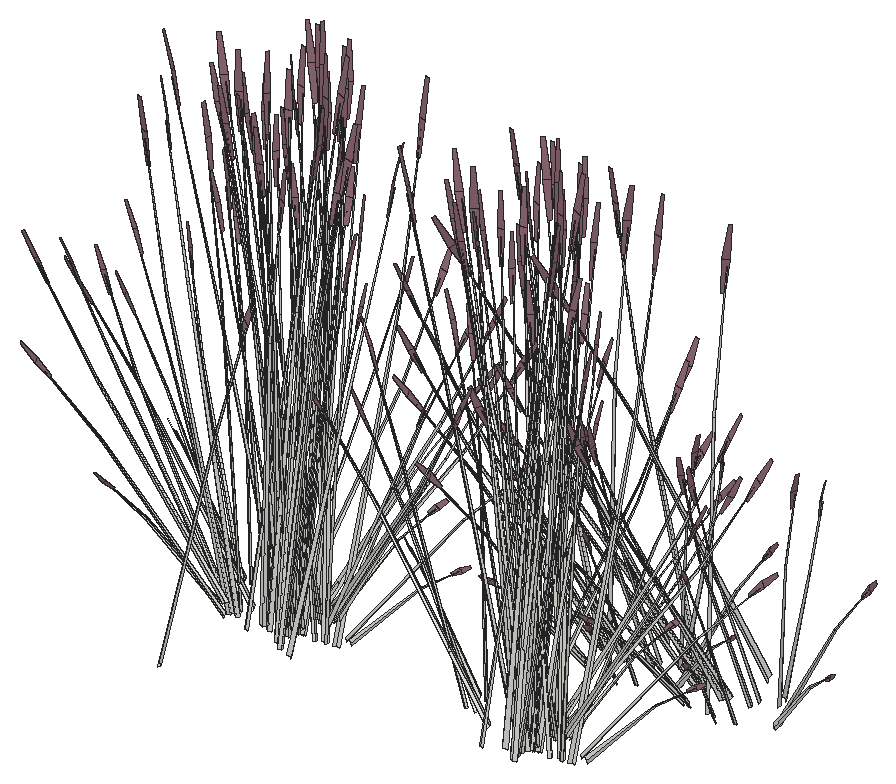
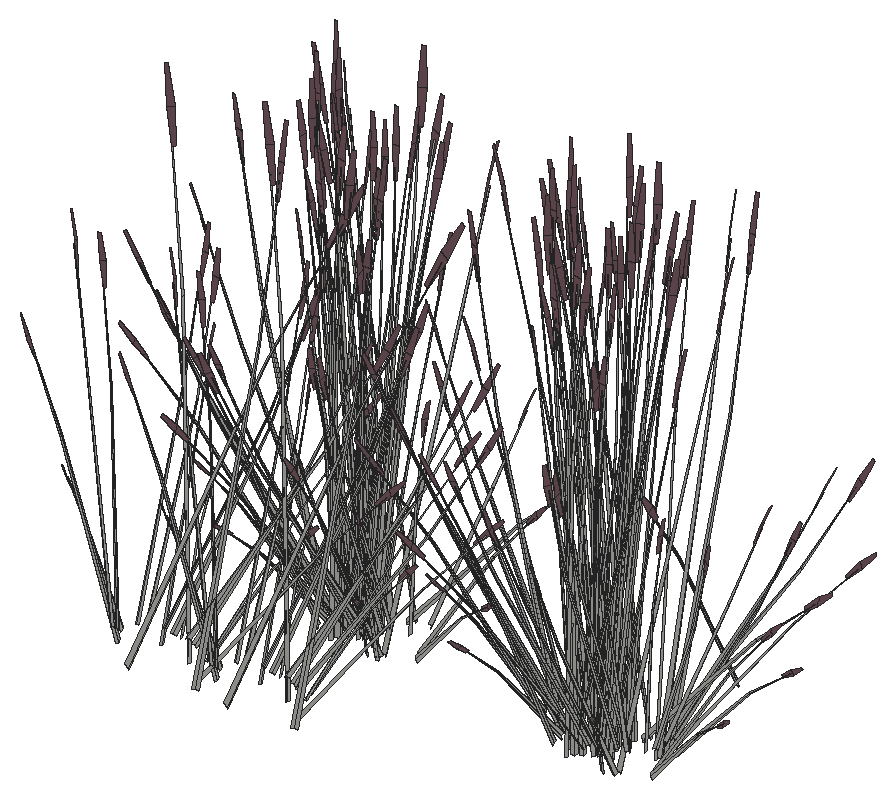
# SketchUp Ruby script. Lengths in inches.
U = 1.inch
M = Sketchup.active_model
def pt(a) = Geom::Point3d.new(a.map { |v| v * U })
def face(e, loops, mat)
  f = e.add_face(loops[0].map { |a| pt(a) })
  loops[1..].each { |l| e.add_face(l.map { |a| pt(a) }).erase! }
  f.material = f.back_material = mat if mat
  f
end
# faces: each face lists its corners as indices into pts; further lists are holes
def faces(e, pts, list, mat = nil) = list.each { |f| face(e, (f[0].is_a?(Array) ? f : [f]).map { |l| l.map { |i| pts[i] } }, mat) }
# xy, xz, yz: faces in a plane at the given z, y or x. An outline is a flat list of corners, or four numbers for a rectangle; further outlines are holes
def ring(l) = l.size == 4 ? [[l[0], l[1]], [l[2], l[1]], [l[2], l[3]], [l[0], l[3]]] : l.each_slice(2).to_a
def flat(e, list, mat, &to3) = list.each { |f| face(e, (f[0].is_a?(Array) ? f : [f]).map { |l| ring(l).map { |u, v| to3.(u, v) } }, mat) }
def xy(e, z, list, mat = nil) = flat(e, list, mat) { |x, y| [x, y, z] }
def xz(e, y, list, mat = nil) = flat(e, list, mat) { |x, z| [x, y, z] }
def yz(e, x, list, mat = nil) = flat(e, list, mat) { |y, z| [x, y, z] }
def lines(e, pts, list) = list.each { |a, b| e.add_line(pt(pts[a]), pt(pts[b])) }
# prism: a flat outline (further loops are holes) pulled along v
def prism(e, loops, v, mat = nil)
  f = face(e, loops, mat); d = Geom::Vector3d.new(v.map { |x| x * U })
  f.pushpull(f.normal.samedirection?(d) ? d.length : -d.length)
end
def box(e, o, s, mat = nil) = prism(e, [[o, [o[0] + s[0], o[1], o[2]], [o[0] + s[0], o[1] + s[1], o[2]], [o[0], o[1] + s[1], o[2]]]], [0, 0, s[2]], mat)
def at(x, y, z, deg = 0) = Geom::Transformation.translation(pt([x, y, z])) * Geom::Transformation.rotation(ORIGIN, Z_AXIS, deg.degrees)
def axes(o, x, y, z) = Geom::Transformation.new([*x, 0, *y, 0, *z, 0, *pt(o).to_a, 1])
def part(name) = M.definitions.add(name)
# library, detail: a bought-in or finely detailed component or shape, given as its bounding box
def library(name, o, s) = part(name).tap { |d| box(d.entities, o, s) }
def detail(e, o, s) = box(e.add_group.entities, o, s)
def put(e, d, t, mat = nil) = e.add_instance(d, t).tap { |i| i.material = mat if mat }
def group(e, t, mat = nil) = e.add_group.tap { |g| g.transformation = t; g.material = mat if mat }.entities
root = M.entities
M.materials.add("LightPink_Translucent").color = [144, 107, 117]
c1 = part("blade")
p = [[2.15,0.21,22],[0,0.17,0],[0.09,0.45,0],[2.18,0.31,22],[2.29,0.31,22],[0.38,0.45,0],
  [2.48,0.24,33],[2.49,0.24,33],[2.48,0.22,33]]
faces(c1.entities,p,[[0,1,2,3],[4,5,2,3],[6,3,4,7],[8,0,3,6]])
c2 = part("seeds")
p = [[0.3,-0.1,1.38],[-0.01,-0.03,1.59],[-0.01,-0.03,0.03],[0.14,-0.07,-0.07],[0.29,-0.03,3],[0.15,0.01,3.11]]
faces(c2.entities,p,[[0,1,2,3],[1,0,4,5]],"LightPink_Translucent")
c3 = part("blade with seeds")
put(c3.entities,c1,at(0,0,0))
put(c3.entities,c2,axes([2.4,0.25,30.99],[1.5799,-0.05474,1.17369],[-0.12525,1.92788,0.29478],[-0.07173,-0.02425,1.56792]))
put(root,c3,axes([68.36,54.11,46.98],[1.07686,-0.45739,-0.71045],[0.60013,0.94154,0.08574],[0.52031,-0.10696,1.00501]))
put(root,c3,axes([63.53,52.48,44.36],[-1.01611,0.93987,0.45755],[-1.20717,-0.82966,0.17955],[0.24496,-0.0938,1.58856]))
put(root,c3,axes([26.46,57.1,44.375],[-1.53239,0,0],[0,-1.1575,-0.51607],[0,-0.26363,1.63711]))
put(root,c3,axes([64.64,54.17,44.3],[-1.1399,-0.8914,-0.06131],[1.1406,-0.89194,0],[-0.03981,-0.03113,1.75571]))
put(root,c3,axes([26.72,55.03,44.59],[0.23927,0.28834,1.43002],[-0.55135,0.78376,-0.30754],[-0.56612,-0.18733,0.61141]))
put(root,c3,axes([61.77,50.93,44.47],[-0.35402,1.02926,0.17642],[-1.29548,-0.29127,0.35086],[0.22379,-0.00501,1.60407]))
put(root,c3,axes([28.39,42.73,45.36],[0.02693,-0.53464,1.54345],[1.21102,0.2824,0.21329],[-0.10493,0.5698,0.72882]))
put(root,c3,axes([64.48,52.08,44.62],[0.23642,-0.92427,0.1448],[1.15506,0.16044,-0.41347],[0.21021,0.09491,1.26744]))
put(root,c3,axes([27.71,54.77,46.98],[-1.22504,-0.02494,-0.71045],[0.08228,-1.05005,0.08574],[-0.51899,-0.11081,1.00501]))
put(root,c3,axes([62.48,54.27,44.36],[1.54892,0.2182,0.45755],[-0.31522,1.23236,0.17955],[-0.22636,-0.119,1.58856]))
put(root,c3,axes([63.98,52.32,44.72],[-0.73619,-0.86927,0.44739],[1.11511,-0.61213,-0.21531],[0.23824,0.10756,1.43643]))
put(root,c3,axes([61.65,56.24,44.47],[1.31687,-0.27488,0.17642],[0.32517,1.02297,0.35086],[-0.11745,-0.14905,1.60407]))
put(root,c3,axes([27.65,56.79,44.33],[-1.1399,0.87071,0.30756],[-1.1406,-0.86155,-0.36492],[-0.03981,-0.24727,1.64885]))
put(root,c3,axes([65.3,53.51,44.21],[1.37109,0,0],[0,1.07219,0],[0,0,1.78407]))
put(root,c3,axes([31.27,57.2,44.43],[1.3808,0.50196,0.24065],[-0.66454,1.04299,0.50002],[0,-0.24043,1.60543]))
put(root,c3,axes([65.6875,50.99,44.47],[-1.31687,0.27488,0.17642],[-0.32517,-1.02297,0.35086],[0.11745,0.14905,1.60407]))
put(root,c3,axes([27.3,54.99,46.68],[-0.88986,0.68603,-0.51099],[-0.77932,-0.72471,-0.3958],[-0.45212,-0.10438,0.97773]))
put(root,c3,axes([25.3,55.9,44.77],[0.78239,-0.07411,1.1486],[-0.49629,0.65296,0.84392],[-0.38663,-0.09795,0.25299]))
put(root,c3,axes([30.83,56.5,44.72],[-1.33077,0.06393,0.44739],[-0.12035,-1.06125,-0.21531],[0.23824,-0.10756,1.43643]))
put(root,c3,axes([27.39,57.27,44.48],[0,1.03566,0.49651],[-1.37109,0,0],[0,-0.23588,1.57504]))
put(root,c3,axes([64.86,52.96,44.38],[-1.54892,-0.2182,0.49198],[0.31522,-1.23236,0.19306],[0.22636,0.119,1.70813]))
put(root,c3,axes([37.02,57.51,46.68],[0.332,-0.94205,-0.51099],[1.13828,0.3229,-0.3958],[0.45829,-0.08638,0.97773]))
put(root,c3,axes([63.62,56,44.2],[-0.39985,-0.89288,0],[1.1418,-0.31268,0],[0,0,1.54371]))
put(root,c3,axes([35.22,53.67,44.375],[0.7662,-1.03778,0],[1.28187,0.57875,-0.51607],[0.29196,0.13181,1.63711]))
put(root,c3,axes([62.86,55.15,44.62],[-0.23642,0.92427,0.1448],[-1.15506,-0.16044,-0.41347],[-0.21021,-0.09491,1.26744]))
put(root,c3,axes([30.78,56.88,44.36],[0.53281,1.15808,0.45755],[-1.52239,0.4027,0.17955],[0.01861,-0.2128,1.58856]))
put(root,c3,axes([65.5625,56.3,44.47],[0.35402,-1.02926,0.17642],[1.29548,0.29127,0.35086],[-0.22379,0.00501,1.60407]))
put(root,c3,axes([65.27,53.96,44.21],[0.85545,0.66896,0],[-0.85545,0.66896,0],[0,0,1.69266]))
put(root,c3,axes([30.51,57.8,44.72],[-0.59459,0.93321,0.44739],[-1.23546,-0.44912,-0.21531],[0,-0.21512,1.43643]))
put(root,c3,axes([60.41,52.71,45.34],[0.34834,-0.14982,1.77064],[0.12012,1.04605,0.13857],[-0.75452,0.1388,0.63284]))
put(root,c3,axes([67.59,53.67,44.47],[-0.96285,-0.75439,0.17642],[0.97031,-0.7317,0.35086],[-0.10634,0.15406,1.60407]))
put(root,c3,axes([32.7,56.98,44.21],[0,-1.19833,0],[1.53239,0,0],[0,0,1.79456]))
put(root,c3,axes([71.4375,54.36,44.77],[-0.75718,0.17097,1.1486],[0.35641,-0.70661,0.84392],[0.40168,0.04835,0.25299]))
put(root,c3,axes([34.56,54.21,44.48],[-1.14694,-0.51783,0.49651],[0.68554,-0.92854,0],[0.26122,0.11794,1.57504]))
put(root,c3,axes([36.8,57.85,46.98],[1.07686,-0.45739,-0.71045],[0.60013,0.94154,0.08574],[0.52031,-0.10696,1.00501]))
put(root,c3,axes([63.34,56.41,44.2],[-1.23546,-0.46496,0],[0.59459,-0.96613,0],[0,0,1.62707]))
put(root,c3,axes([61.22,56.77,44.48],[1.14694,0.51783,0.49651],[-0.68554,0.92854,0],[-0.26122,-0.11794,1.57504]))
put(root,c3,axes([31.97,56.23,44.36],[-1.01611,0.93987,0.45755],[-1.20717,-0.82966,0.17955],[0.24496,-0.0938,1.58856]))
put(root,c3,axes([65.26,53.18,44.72],[0.59459,-0.93321,0.44739],[1.23546,0.44912,-0.21531],[0,0.21512,1.43643]))
put(root,c3,axes([33.08,57.91,44.3],[-1.1399,-0.8914,-0.06131],[1.1406,-0.89194,0],[-0.03981,-0.03113,1.75571]))
put(root,c3,axes([30.21,54.68,44.47],[-0.35402,1.02926,0.17642],[-1.29548,-0.29127,0.35086],[0.22379,-0.00501,1.60407]))
put(root,c3,axes([65.03,53.72,44.29],[0,1.19774,-0.05637],[-1.53239,0,0],[0,0.03764,1.79368]))
put(root,c3,axes([58,53.28,46.68],[-0.332,0.94205,-0.51099],[-1.13828,-0.3229,-0.3958],[-0.45829,0.08638,0.97773]))
put(root,c3,axes([32.91,55.82,44.62],[0.23642,-0.92427,0.1448],[1.15506,0.16044,-0.41347],[0.21021,0.09491,1.26744]))
put(root,c3,axes([60.56,57.31,44.375],[-0.7662,1.03778,0],[-1.28187,-0.57875,-0.51607],[-0.29196,-0.13181,1.63711]))
put(root,c3,axes([30.92,58.02,44.36],[1.54892,0.2182,0.45755],[-0.31522,1.23236,0.17955],[-0.22636,-0.119,1.58856]))
put(root,c3,axes([68.38,53.7,44.48],[0,-1.03566,0.49651],[1.37109,0,0],[0,0.23588,1.57504]))
put(root,c3,axes([64.94,54.48,44.72],[1.33077,-0.06393,0.44739],[0.12035,1.06125,-0.21531],[-0.23824,0.10756,1.43643]))
put(root,c3,axes([65.77,53.4,44.62],[1.1418,-0.30203,0.1448],[0.39985,0.86246,-0.41347],[0,0.18981,1.26744]))
put(root,c3,axes([32.42,56.07,44.72],[-0.73619,-0.86927,0.44739],[1.11511,-0.61213,-0.21531],[0.23824,0.10756,1.43643]))
put(root,c3,axes([70.02,55.5,44.59],[-0.29514,-0.25472,1.43002],[0.38401,-0.84262,-0.30754],[0.59714,0.11414,0.61141]))
put(root,c3,axes([30.08,59.99,44.47],[1.31687,-0.27488,0.17642],[0.32517,1.02297,0.35086],[-0.11745,-0.14905,1.60407]))
put(root,c3,axes([37.71,57.94,46.53],[1.01846,0.28891,-0.35414],[-0.29705,0.84289,0.4572],[0.41005,-0.07729,0.87481]))
put(root,c3,axes([64.74,56.42,44.2],[1.23546,0.46496,0],[-0.59459,0.96613,0],[0,0,1.74954]))
put(root,c3,axes([25.74,56.59,46.53],[-1.01846,-0.28891,-0.35414],[0.29705,-0.84289,0.4572],[-0.41005,0.07729,0.87481]))
put(root,c3,axes([33.74,57.25,44.21],[1.37109,0,0],[0,1.07219,0],[0,0,1.78407]))
put(root,c3,axes([34.125,54.73,44.47],[-1.31687,0.27488,0.17642],[-0.32517,-1.02297,0.35086],[0.11745,0.14905,1.60407]))
put(root,c3,axes([65.23,57.45,44.19],[-0.75665,-1.04141,-0.05142],[1.28187,-0.57875,0.51607],[-0.31588,0.09915,1.6363]))
put(root,c3,axes([64.97,54.93,44.62],[0.90538,0.62224,0.1448],[-0.75521,0.70202,-0.41347],[-0.21021,0.09491,1.26744]))
put(root,c3,axes([67.31,56.01,46.98],[1.22504,0.02494,-0.71045],[-0.08228,1.05005,0.08574],[0.51899,0.11081,1.00501]))
put(root,c3,axes([33.29,56.7,44.38],[-1.54892,-0.2182,0.49198],[0.31522,-1.23236,0.19306],[0.22636,0.119,1.70813]))
put(root,c3,axes([32.06,59.75,44.2],[-0.39985,-0.89288,0],[1.1418,-0.31268,0],[0,0,1.54371]))
put(root,c3,axes([65.93,56.85,44.48],[1.14694,-0.51783,0.49651],[0.68554,0.92854,0],[-0.26122,0.11794,1.57504]))
put(root,c3,axes([31.3,58.9,44.62],[-0.23642,0.92427,0.1448],[-1.15506,-0.16044,-0.41347],[-0.21021,-0.09491,1.26744]))
put(root,c3,axes([64.3,56.03,44.29],[0.53281,1.18979,-0.06012],[-1.52239,0.41691,0],[0.01861,0.04155,1.72173]))
put(root,c3,axes([34,60.04,44.47],[0.35402,-1.02926,0.17642],[1.29548,0.29127,0.35086],[-0.22379,0.00501,1.60407]))
put(root,c3,axes([56.64,55.49,44.59],[0.42589,0.08502,1.43002],[0.2745,0.86839,-0.30754],[-0.57851,0.16255,0.61141]))
put(root,c3,axes([33.71,57.71,44.21],[0.85545,0.66896,0],[-0.85545,0.66896,0],[0,0,1.69266]))
put(root,c3,axes([69.31,53.88,44.375],[1.53239,0,0],[0,1.1575,-0.51607],[0,0.26363,1.63711]))
put(root,c3,axes([28.84,56.45,45.34],[0.34834,-0.14982,1.77064],[0.12012,1.04605,0.13857],[-0.75452,0.1388,0.63284]))
put(root,c3,axes([36.02,57.42,44.47],[-0.96285,-0.75439,0.17642],[0.97031,-0.7317,0.35086],[-0.10634,0.15406,1.60407]))
put(root,c3,axes([68.7,54.47,44.2],[-1.53164,-0.00828,-0.04976],[0,-1.1575,0.49943],[-0.04813,0.2635,1.58352]))
put(root,c3,axes([39.875,58.11,44.77],[-0.75718,0.17097,1.1486],[0.35641,-0.70661,0.84392],[0.40168,0.04835,0.25299]))
put(root,c3,axes([55.75,57.31,44.77],[0.51072,-0.46938,1.1486],[0.20153,0.74307,0.84392],[-0.36908,0.13305,0.25299]))
put(root,c3,axes([68.05,56.44,46.53],[0.69728,0.64842,-0.35414],[-0.79619,0.61382,0.4572],[0.40453,0.09339,0.87481]))
put(root,c3,axes([31.78,60.15,44.2],[-1.23546,-0.46496,0],[0.59459,-0.96613,0],[0,0,1.62707]))
put(root,c3,axes([29.65,60.51,44.48],[1.14694,0.51783,0.49651],[-0.68554,0.92854,0],[-0.26122,-0.11794,1.57504]))
put(root,c3,axes([33.7,56.93,44.72],[0.59459,-0.93321,0.44739],[1.23546,0.44912,-0.21531],[0,0.21512,1.43643]))
put(root,c3,axes([33.47,57.46,44.29],[0,1.19774,-0.05637],[-1.53239,0,0],[0,0.03764,1.79368]))
put(root,c3,axes([26.44,57.02,46.68],[-0.332,0.94205,-0.51099],[-1.13828,-0.3229,-0.3958],[-0.45829,0.08638,0.97773]))
put(root,c3,axes([28.99,61.05,44.375],[-0.7662,1.03778,0],[-1.28187,-0.57875,-0.51607],[-0.29196,-0.13181,1.63711]))
put(root,c3,axes([36.82,57.45,44.48],[0,-1.03566,0.49651],[1.37109,0,0],[0,0.23588,1.57504]))
put(root,c3,axes([33.38,58.22,44.72],[1.33077,-0.06393,0.44739],[0.12035,1.06125,-0.21531],[-0.23824,0.10756,1.43643]))
put(root,c3,axes([34.21,57.14,44.62],[1.1418,-0.30203,0.1448],[0.39985,0.86246,-0.41347],[0,0.18981,1.26744]))
put(root,c3,axes([65.27,56.92,44.33],[1.53422,0.33662,0.30756],[-0.38383,1.20322,-0.36492],[-0.25393,0.15059,1.64885]))
put(root,c3,axes([38.46,59.24,44.59],[-0.29514,-0.25472,1.43002],[0.38401,-0.84262,-0.30754],[0.59714,0.11414,0.61141]))
put(root,c3,axes([67.23,56.8125,44.77],[-0.69001,-0.29779,1.1486],[0.89096,-0.30257,0.84392],[0.24031,0.2563,0.25299]))
put(root,c3,axes([33.18,60.17,44.2],[1.23546,0.46496,0],[-0.59459,0.96613,0],[0,0,1.74954]))
put(root,c3,axes([33.67,61.2,44.19],[-0.75665,-1.04141,-0.05142],[1.28187,-0.57875,0.51607],[-0.31588,0.09915,1.6363]))
put(root,c3,axes([58.56,55.38,46.68],[0.31482,0.94565,-0.51099],[-1.19224,0.16542,-0.3958],[-0.34166,0.254,0.97773]))
put(root,c3,axes([33.4,58.68,44.62],[0.90538,0.62224,0.1448],[-0.75521,0.70202,-0.41347],[-0.21021,0.09491,1.26744]))
put(root,c3,axes([65.625,69.54,44.59],[-0.34835,0.20963,1.43002],[-1.04325,-0.36691,-0.30754],[0.19338,-0.4563,0.61141]))
put(root,c3,axes([77.625,69.54,44.59],[-0.34835,0.20963,1.43002],[-1.04325,-0.36691,-0.30754],[0.19338,-0.4563,0.61141]))
put(root,c3,axes([66.2,57.57,44.375],[0.7662,1.03778,0],[-1.28187,0.57875,-0.51607],[-0.29196,0.13181,1.63711]))
put(root,c3,axes([64.04,70.27,46.98],[-0.5849,-0.8421,-0.71045],[1.20401,-0.4693,0.08574],[-0.13677,-0.40688,1.00501]))
put(root,c3,axes([76.04,70.27,46.98],[-0.5849,-0.8421,-0.71045],[1.20401,-0.4693,0.08574],[-0.13677,-0.40688,1.00501]))
put(root,c3,axes([60.23,69.14,44.59],[-0.07421,0.33879,1.43002],[-1.08488,0.28361,-0.30754],[-0.25359,-0.4379,0.61141]))
put(root,c3,axes([72.23,69.14,44.59],[-0.07421,0.33879,1.43002],[-1.08488,0.28361,-0.30754],[-0.25359,-0.4379,0.61141]))
put(root,c3,axes([65.55,53.46,44.84],[-0.03348,-0.97511,1.41272],[1.51511,0.25277,0.59816],[-0.35835,0.53357,1.3335]))
put(root,c3,axes([65.67,57.22,46.68],[1.20928,-0.24619,-0.51099],[0.21154,0.93233,-0.3958],[0.32481,0.26718,0.97773]))
put(root,c3,axes([35.75,59.75,46.98],[1.22504,0.02494,-0.71045],[-0.08228,1.05005,0.08574],[0.51899,0.11081,1.00501]))
put(root,c3,axes([34.37,60.59,44.48],[1.14694,-0.51783,0.49651],[0.68554,0.92854,0],[-0.26122,0.11794,1.57504]))
put(root,c3,axes([32.74,59.78,44.29],[0.53281,1.18979,-0.06012],[-1.52239,0.41691,0],[0.01861,0.04155,1.72173]))
put(root,c3,axes([66.47,71.09,46.98],[0.03189,-0.95798,-0.71045],[1.34277,0.06434,0.08574],[0.14171,-0.40585,1.00501]))
put(root,c3,axes([78.47,71.09,46.98],[0.03189,-0.95798,-0.71045],[1.34277,0.06434,0.08574],[0.14171,-0.40585,1.00501]))
put(root,c3,axes([67.34,58.17,44.67],[-0.78586,-0.03248,1.0506],[0.51898,-0.68985,0.58006],[0.31045,0.24509,0.8241]))
put(root,c3,axes([25.08,59.23,44.59],[0.42589,0.08502,1.43002],[0.2745,0.86839,-0.30754],[-0.57851,0.16255,0.61141]))
put(root,c3,axes([37.75,57.62,44.375],[1.53239,0,0],[0,1.1575,-0.51607],[0,0.26363,1.63711]))
put(root,c3,axes([37.14,58.22,44.2],[-1.53164,-0.00828,-0.04976],[0,-1.1575,0.49943],[-0.04813,0.2635,1.58352]))
put(root,c3,axes([24.19,61.05,44.77],[0.51072,-0.46938,1.1486],[0.20153,0.74307,0.84392],[-0.36908,0.13305,0.25299]))
put(root,c3,axes([36.48,60.1875,46.53],[0.69728,0.64842,-0.35414],[-0.79619,0.61382,0.4572],[0.40453,0.09339,0.87481]))
put(root,c3,axes([63.6,70.1,46.68],[-1.20468,-0.25962,-0.51099],[0.41292,-0.89013,-0.3958],[-0.11046,-0.35838,0.97773]))
put(root,c3,axes([75.6,70.1,46.68],[-1.20468,-0.25962,-0.51099],[0.41292,-0.89013,-0.3958],[-0.11046,-0.35838,0.97773]))
put(root,c3,axes([64.34,67.87,44.77],[0.15721,0.60392,1.1486],[-0.87211,-0.33448,0.84392],[0.09385,-0.30923,0.25299]))
put(root,c3,axes([76.34,67.87,44.77],[0.15721,0.60392,1.1486],[-0.87211,-0.33448,0.84392],[0.09385,-0.30923,0.25299]))
put(root,c3,axes([26.12,59.02,46.53],[-1.06674,0.14801,-0.35414],[-0.28168,-0.84611,0.4572],[-0.30569,0.22726,0.87481]))
put(root,c3,axes([66.2,70.77,46.68],[-0.87728,-0.69587,-0.51099],[0.92674,-0.60943,-0.3958],[0.13348,-0.35356,0.97773]))
put(root,c3,axes([78.2,70.77,46.68],[-0.87728,-0.69587,-0.51099],[0.92674,-0.60943,-0.3958],[0.13348,-0.35356,0.97773]))
put(root,c3,axes([64.77,56.49,44.59],[0.02163,-0.34331,1.43002],[1.03345,-0.38348,-0.30754],[0.31903,0.4109,0.61141]))
put(root,c3,axes([60.08,59.36,44.77],[-0.03171,-0.6158,1.1486],[0.7925,0.43922,0.84392],[-0.15586,0.29352,0.25299]))
put(root,c3,axes([33.71,60.66,44.33],[1.53422,0.33662,0.30756],[-0.38383,1.20322,-0.36492],[-0.25393,0.15059,1.64885]))
put(root,c3,axes([59.86,68.6,44.77],[0.63926,0.36046,1.1486],[-0.93099,0.21668,0.84392],[-0.1992,-0.27702,0.25299]))
put(root,c3,axes([71.86,68.6,44.77],[0.63926,0.36046,1.1486],[-0.93099,0.21668,0.84392],[-0.1992,-0.27702,0.25299]))
put(root,c3,axes([61.4,70.51,46.98],[-1.04497,-0.50058,-0.71045],[0.74264,-0.8772,0.08574],[-0.3786,-0.29889,1.00501]))
put(root,c3,axes([73.4,70.51,46.98],[-1.04497,-0.50058,-0.71045],[0.74264,-0.8772,0.08574],[-0.3786,-0.29889,1.00501]))
put(root,c3,axes([60.38,56.98,47],[0.87728,0.69587,-0.5672],[-0.92674,0.60943,-0.43934],[-0.13348,0.35356,1.08528]))
put(root,c3,axes([59.43,58.03,44.82],[1.11329,-0.1834,0.06507],[0.25594,0.73887,-0.86304],[-0.07058,0.37403,0.7736]))
put(root,c3,axes([62.98,57.66,46.68],[1.20468,0.25962,-0.51099],[-0.41292,0.89013,-0.3958],[0.11046,0.35838,0.97773]))
put(root,c3,axes([35.66,60.56,44.77],[-0.69001,-0.29779,1.1486],[0.89096,-0.30257,0.84392],[0.24031,0.2563,0.25299]))
put(root,c3,axes([27,59.12,46.68],[0.31482,0.94565,-0.51099],[-1.19224,0.16542,-0.3958],[-0.34166,0.254,0.97773]))
put(root,c3,axes([34.64,61.3125,44.375],[0.7662,1.03778,0],[-1.28187,0.57875,-0.51607],[-0.29196,0.13181,1.63711]))
put(root,c3,axes([60.11,56.66,47.34],[-0.03189,0.95798,-0.7886],[-1.34277,-0.06434,0.09517],[-0.14171,0.40585,1.11556]))
put(root,c3,axes([33.98,57.2,44.84],[-0.03348,-0.97511,1.41272],[1.51511,0.25277,0.59816],[-0.35835,0.53357,1.3335]))
put(root,c3,axes([34.11,60.97,46.68],[1.20928,-0.24619,-0.51099],[0.21154,0.93233,-0.3958],[0.32481,0.26718,0.97773]))
put(root,c3,axes([60.91,70.53,46.68],[-1.20928,0.24619,-0.51099],[-0.21154,-0.93233,-0.3958],[-0.32481,-0.26718,0.97773]))
put(root,c3,axes([72.91,70.53,46.68],[-1.20928,0.24619,-0.51099],[-0.21154,-0.93233,-0.3958],[-0.32481,-0.26718,0.97773]))
put(root,c3,axes([35.77,61.91,44.67],[-0.78586,-0.03248,1.0506],[0.51898,-0.68985,0.58006],[0.31045,0.24509,0.8241]))
put(root,c3,axes([62.54,57.49,46.98],[0.5849,0.8421,-0.71045],[-1.20401,0.4693,0.08574],[0.13677,0.40688,1.00501]))
put(root,c3,axes([68.06,72.76,46.98],[0.64013,-0.81717,-0.71045],[1.12174,0.58074,0.08574],[0.38221,-0.29607,1.00501]))
put(root,c3,axes([80.06,72.76,46.98],[0.64013,-0.81717,-0.71045],[1.12174,0.58074,0.08574],[0.38221,-0.29607,1.00501]))
put(root,c3,axes([61.14,70.38,44.375],[-0.7662,-1.03778,0],[1.28187,-0.57875,-0.51607],[0.29196,-0.13181,1.63711]))
put(root,c3,axes([73.14,70.38,44.375],[-0.7662,-1.03778,0],[1.28187,-0.57875,-0.51607],[0.29196,-0.13181,1.63711]))
put(root,c3,axes([68.02,72.375,46.68],[-0.31482,-0.94565,-0.51099],[1.19224,-0.16542,-0.3958],[0.34166,-0.254,0.97773]))
put(root,c3,axes([80.02,72.375,46.68],[-0.31482,-0.94565,-0.51099],[1.19224,-0.16542,-0.3958],[0.34166,-0.254,0.97773]))
put(root,c3,axes([59.16,58.81,44.59],[0.38672,-0.16338,1.43002],[0.95481,0.49262,-0.30754],[-0.28419,0.42626,0.61141]))
put(root,c3,axes([33.21,60.24,44.59],[0.02163,-0.34331,1.43002],[1.03345,-0.38348,-0.30754],[0.31903,0.4109,0.61141]))
put(root,c3,axes([63.9,76.17,45.33],[1.05902,0.41762,1.51261],[-1.03748,0.89969,0.59816],[-0.46471,-0.53324,1.26806]))
put(root,c3,axes([75.9,76.17,45.33],[1.05902,0.41762,1.51261],[-1.03748,0.89969,0.59816],[-0.46471,-0.53324,1.26806]))
put(root,c3,axes([27.99,60.98,46.53],[-0.82919,0.54528,-0.35414],[-0.78493,-0.62262,0.4572],[-0.11943,0.31634,0.87481]))
put(root,c3,axes([68.98,72.01,44.59],[-0.4378,-0.03068,1.43002],[-0.44851,-0.8229,-0.30754],[0.53783,-0.23279,0.61141]))
put(root,c3,axes([80.98,72.01,44.59],[-0.4378,-0.03068,1.43002],[-0.44851,-0.8229,-0.30754],[0.53783,-0.23279,0.61141]))
put(root,c3,axes([59.66,58.01,45.36],[0.02693,-0.53464,1.54345],[1.21102,0.2824,0.21329],[-0.10493,0.5698,0.72882]))
put(root,c3,axes([28.52,63.1,44.77],[-0.03171,-0.6158,1.1486],[0.7925,0.43922,0.84392],[-0.15586,0.29352,0.25299]))
put(root,c3,axes([69.49,70.49,44.77],[-0.40819,0.5272,1.1486],[-0.35086,-0.70831,0.84392],[0.33713,-0.17749,0.25299]))
put(root,c3,axes([81.49,70.49,44.77],[-0.40819,0.5272,1.1486],[-0.35086,-0.70831,0.84392],[0.33713,-0.17749,0.25299]))
put(root,c3,axes([28.82,60.72,47],[0.87728,0.69587,-0.5672],[-0.92674,0.60943,-0.43934],[-0.13348,0.35356,1.08528]))
put(root,c3,axes([27.87,61.77,44.82],[1.11329,-0.1834,0.06507],[0.25594,0.73887,-0.86304],[-0.07058,0.37403,0.7736]))
put(root,c3,axes([31.42,61.4,46.68],[1.20468,0.25962,-0.51099],[-0.41292,0.89013,-0.3958],[0.11046,0.35838,0.97773]))
put(root,c3,axes([30.87,61.94,46.53],[-0.36946,0.79643,-0.35414],[-1.07787,-0.23229,0.4572],[0.09883,0.32066,0.87481]))
put(root,c3,axes([58.02,74.07,44.375],[-1.53239,0,0],[0,-1.1575,-0.51607],[0,-0.26363,1.63711]))
put(root,c3,axes([70.02,74.07,44.375],[-1.53239,0,0],[0,-1.1575,-0.51607],[0,-0.26363,1.63711]))
put(root,c3,axes([28.55,60.41,47.34],[-0.03189,0.95798,-0.7886],[-1.34277,-0.06434,0.09517],[-0.14171,0.40585,1.11556]))
put(root,c3,axes([58.29,72,44.59],[0.23927,0.28834,1.43002],[-0.55135,0.78376,-0.30754],[-0.56612,-0.18733,0.61141]))
put(root,c3,axes([70.29,72,44.59],[0.23927,0.28834,1.43002],[-0.55135,0.78376,-0.30754],[-0.56612,-0.18733,0.61141]))
put(root,c3,axes([59.27,71.75,46.98],[-1.22504,-0.02494,-0.71045],[0.08228,-1.05005,0.08574],[-0.51899,-0.11081,1.00501]))
